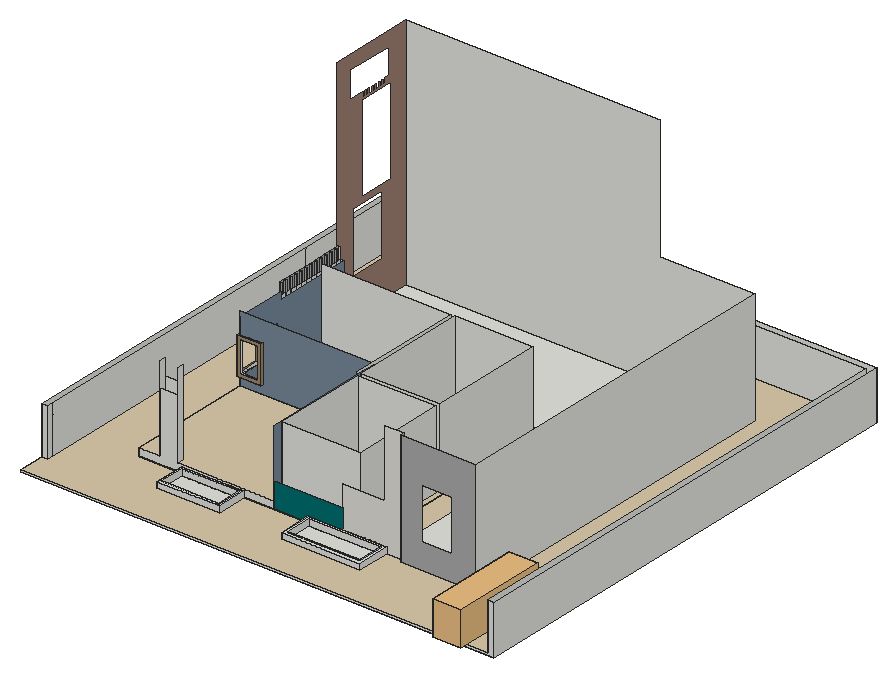
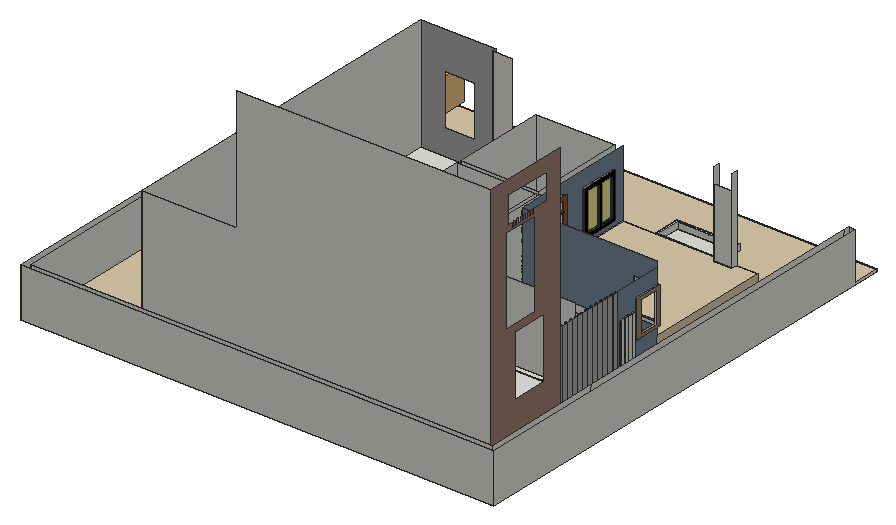
# SketchUp Ruby script. Lengths in inches.
U = 1.inch
M = Sketchup.active_model
def pt(a) = Geom::Point3d.new(a.map { |v| v * U })
def face(e, loops, mat)
  f = e.add_face(loops[0].map { |a| pt(a) })
  loops[1..].each { |l| e.add_face(l.map { |a| pt(a) }).erase! }
  f.material = f.back_material = mat if mat
  f
end
# faces: each face lists its corners as indices into pts; further lists are holes
def faces(e, pts, list, mat = nil) = list.each { |f| face(e, (f[0].is_a?(Array) ? f : [f]).map { |l| l.map { |i| pts[i] } }, mat) }
# xy, xz, yz: faces in a plane at the given z, y or x. An outline is a flat list of corners, or four numbers for a rectangle; further outlines are holes
def ring(l) = l.size == 4 ? [[l[0], l[1]], [l[2], l[1]], [l[2], l[3]], [l[0], l[3]]] : l.each_slice(2).to_a
def flat(e, list, mat, &to3) = list.each { |f| face(e, (f[0].is_a?(Array) ? f : [f]).map { |l| ring(l).map { |u, v| to3.(u, v) } }, mat) }
def xy(e, z, list, mat = nil) = flat(e, list, mat) { |x, y| [x, y, z] }
def xz(e, y, list, mat = nil) = flat(e, list, mat) { |x, z| [x, y, z] }
def yz(e, x, list, mat = nil) = flat(e, list, mat) { |y, z| [x, y, z] }
def lines(e, pts, list) = list.each { |a, b| e.add_line(pt(pts[a]), pt(pts[b])) }
# prism: a flat outline (further loops are holes) pulled along v
def prism(e, loops, v, mat = nil)
  f = face(e, loops, mat); d = Geom::Vector3d.new(v.map { |x| x * U })
  f.pushpull(f.normal.samedirection?(d) ? d.length : -d.length)
end
def box(e, o, s, mat = nil) = prism(e, [[o, [o[0] + s[0], o[1], o[2]], [o[0] + s[0], o[1] + s[1], o[2]], [o[0], o[1] + s[1], o[2]]]], [0, 0, s[2]], mat)
def at(x, y, z, deg = 0) = Geom::Transformation.translation(pt([x, y, z])) * Geom::Transformation.rotation(ORIGIN, Z_AXIS, deg.degrees)
def axes(o, x, y, z) = Geom::Transformation.new([*x, 0, *y, 0, *z, 0, *pt(o).to_a, 1])
def part(name) = M.definitions.add(name)
# library, detail: a bought-in or finely detailed component or shape, given as its bounding box
def library(name, o, s) = part(name).tap { |d| box(d.entities, o, s) }
def detail(e, o, s) = box(e.add_group.entities, o, s)
def put(e, d, t, mat = nil) = e.add_instance(d, t).tap { |i| i.material = mat if mat }
def group(e, t, mat = nil) = e.add_group.tap { |g| g.transformation = t; g.material = mat if mat }.entities
root = M.entities
M.materials.add("Niraj_Skin").color = [158, 128, 115]
M.materials.add("[0035_Tan]").color = [158, 135, 105]
M.materials.add("[0110_LightSlateGray]").color = [119, 136, 153]
M.materials.add("[Color H07]1").color = [0, 109, 109]
M.materials.add("[Color M03]").color = [170, 170, 170]
M.materials.add("[Color M09]").color = [0, 0, 0]
M.materials.add("[Field Square Tile]").color = [217, 201, 169]
M.materials.add("[Marble Carrara Gold Floor Tile]").color = [225, 223, 217]
M.materials.add("[Translucent Glass Gray]").color = [242, 225, 74]
M.materials["[Translucent Glass Gray]"].alpha = 0.5
M.materials.add("[Wood Cherry Original]").color = [152, 86, 42]
c1 = library("Potted plant collection",[-0.05,-0.05,0],[59.02,14.54,22.0625])
xy(root,12.61,[[[0,0,720.33,531.02],[89.54,112.91,428.79,458.91]],[89.54,112.91,89.54,266.1,98.54,266.1,98.54,121.91,294.79,121.91,294.79,112.91],[[294.79,112.91,294.79,266.1,89.54,266.1,89.54,458.91,428.79,458.91,428.79,112.91],[98.54,272.1,294.79,449.91],[300.79,272.1,419.79,449.91],[300.79,121.91,419.79,266.1]],[98.54,121.91,294.79,266.1],[300.79,121.91,419.79,266.1],
  [98.54,272.1,294.79,449.91],[300.79,272.1,419.79,449.91],[0,531.02,720.33,727.14]])
xy(root,15.11,[[98.54,121.91,98.54,305.6,294.79,305.6,294.79,286.89,288.79,286.89,288.79,280.89,291.79,280.89,291.79,260.11,288.79,260.11,288.79,257.5625,291.79,257.5625,291.79,233.45,288.79,233.45,288.79,227.45,294.79,227.45,294.79,121.91]])
xy(root,15.61,[[[347.53,62.1,467.15,112.91],[352.75,67.33,461.93,107.69]],[[154.8,66.73,250.05,112.91],[158.93,70.86,245.92,108.78]],[352.75,67.33,461.93,107.69],[158.93,70.86,245.92,108.78],[493.41,106.91,607.41,106.91,607.41,636.48,463.41,636.48,463.41,112.91,493.41,112.91],
  [294.79,112.91,428.79,112.91,428.79,458.91,89.54,458.91,89.54,305.6,294.79,305.6],[89.54,112.91,98.54,266.1],[98.54,112.91,121.875,121.91],[121.875,112.91,149.09,121.91],[149.09,112.91,294.79,121.91],
  [428.79,112.91,463.41,458.91],[288.79,227.45,294.79,233.45],[291.79,233.45,294.79,266.1],[288.79,257.5625,291.79,260.11],[89.54,266.1,98.54,305.6],
  [291.79,266.1,294.79,272.1],[291.79,272.1,294.79,280.89],[288.79,280.89,294.79,286.89],[86.54,350.68,89.54,354.7],[86.54,357.49,89.54,361.52],
  [86.54,364.68,89.54,368.7],[86.54,371.93,89.54,375.95],[89.54,458.91,463.41,458.91,463.41,636.48,77.54,636.48,77.54,504.04,89.54,504.04]])
xy(root,15.61,[[[0,0,711.33,0,711.33,718.14,9,718.14,9,40.8125,0,40.8125],[347.53,62.1,347.53,112.91,463.41,112.91,463.41,458.91,89.54,458.91,89.54,504.04,77.54,504.04,77.54,636.48,607.41,636.48,607.41,106.91,493.41,106.91,493.41,112.91,467.15,112.91,467.15,62.1],[154.8,66.73,250.05,112.91],[89.54,112.91,89.54,305.6,98.54,305.6,98.54,121.91,149.09,121.91,149.09,112.91],[81.04,392.11,84.04,398.71],[81.04,401.68,84.04,408.27],[81.04,411.24,84.04,417.84],[81.04,420.8,84.04,427.4],[81.04,430.36,84.04,436.96],[81.04,439.93,84.04,446.52],[81.04,449.49,84.04,456.09],[81.04,459.05,84.04,465.65],[81.04,468.61,84.04,475.21],[81.04,478.18,84.04,484.77],[81.04,487.86,84.04,494.46],[81.04,496.61,84.04,503.21],[86.54,350.68,89.54,354.7],[86.54,357.49,89.54,361.52],[86.54,364.68,89.54,368.7],[86.54,371.93,89.54,375.95]]],"[Field Square Tile]")
xy(root,23.13,[[288.79,233.45,291.79,257.5625],[288.79,260.11,291.79,280.89]])
xy(root,24.61,[[[347.53,62.1,467.15,112.91],[352.75,67.33,461.93,107.69]],[[154.8,66.73,250.05,112.91],[158.93,70.86,245.92,108.78]]])
xy(root,24.97,[[288.79,233.45,291.79,257.5625],[288.79,260.11,291.79,280.89]])
xy(root,27.61,[[89.54,112.91,121.875,112.91,121.875,121.91,149.09,121.91,149.09,112.91,294.79,112.91,294.79,227.45,288.79,227.45,288.79,233.45,291.79,233.45,291.79,257.5625,288.79,257.5625,288.79,260.11,291.79,260.11,291.79,280.89,288.79,280.89,288.79,286.89,294.79,286.89,294.79,305.6,89.54,305.6]],"[Field Square Tile]")
xy(root,36.97,[[291.79,131.57,294.79,189.85]])
xy(root,40.7,[[288.79,233.45,291.79,257.5625],[288.79,260.11,291.79,280.89]],"[Color M09]")
xy(root,40.99,[[86.54,302.6,86.54,346.85,89.54,346.85,89.54,305.6,123.91,305.6,123.91,302.6]])
xy(root,42.14,[[291.79,136.74,294.79,157.71],[291.79,160.71,294.79,184.67]],"[Color M09]")
xy(root,42.53,[[288.79,233.45,291.79,257.5625],[288.79,260.11,291.79,280.89]],"[Color M09]")
xz(root,0,[[0,12.61,720.33,12.61,720.33,87.61,711.33,87.61,711.33,15.61,0,15.61]])
xz(root,40.8125,[[0,15.61,9,87.61]])
xz(root,62.1,[[347.53,15.61,467.15,24.61]])
xz(root,66.73,[[154.8,15.61,250.05,24.61]])
xz(root,67.33,[[352.75,15.61,461.93,24.61]])
xz(root,70.86,[[158.93,15.61,245.92,24.61]])
xz(root,106.91,[[[493.41,15.61,607.41,188.93],[524.95,53.97,524.95,131.79,571.26,131.79,571.26,128.66,571.13,128.66,571.13,53.97]]],"[Color M03]")
xz(root,107.69,[[352.75,15.61,461.93,24.61]])
xz(root,108.78,[[158.93,15.61,245.92,24.61]])
xz(root,112.91,[[89.54,12.61,294.79,15.61],[294.79,12.61,428.79,15.61],[89.54,15.61,154.8,15.61,154.8,24.61,250.05,24.61,250.05,15.61,294.79,15.61,294.79,27.61,149.09,27.61,149.09,120.61,121.875,120.61,121.875,27.61,89.54,27.61],[154.8,15.61,250.05,24.61],[347.53,15.61,400.27,24.61],
  [400.27,15.61,428.79,24.61],[428.79,15.61,463.41,24.61],[463.41,15.61,467.15,24.61]])
xz(root,112.91,[[294.79,15.61,347.53,15.61,347.53,24.61,400.27,24.61,400.27,54.34,294.79,54.34]],"[Color H07]1")
xz(root,112.91,[[467.15,15.61,493.41,15.61,493.41,188.93,463.41,188.93,463.41,86.53,400.27,86.53,400.27,24.61,467.15,24.61]],"[Marble Carrara Gold Floor Tile]")
xz(root,121.91,[[98.54,12.61,121.875,15.11],[121.875,12.61,149.09,15.11],[149.09,12.61,294.79,15.11],[300.79,12.61,419.79,132.61],[98.54,15.11,121.875,15.61],
  [121.875,15.11,149.09,15.61],[149.09,15.11,294.79,15.61],[121.875,15.61,149.09,27.61],[121.875,27.61,149.09,132.61]])
xz(root,131.57,[[291.79,36.97,294.79,105.75]],"[Color M09]")
xz(root,136.74,[[291.79,42.14,294.79,100.57]],"[Color M09]")
xz(root,157.71,[[291.79,42.14,294.79,100.57]],"[Color M09]")
xz(root,160.71,[[291.79,42.14,294.79,100.57]],"[Color M09]")
xz(root,184.67,[[291.79,42.14,294.79,100.57]],"[Color M09]")
xz(root,189.85,[[291.79,36.97,294.79,105.75]],"[Color M09]")
xz(root,227.45,[[288.79,15.11,294.79,15.61],[288.79,15.61,294.79,27.61]])
xz(root,227.45,[[288.79,27.61,294.79,115.36]],"[Wood Cherry Original]")
xz(root,233.45,[[288.79,15.11,291.79,15.61],[288.79,15.61,291.79,23.13],[291.79,15.61,294.79,109.36],[288.79,23.13,291.79,24.97],[288.79,24.97,291.79,27.61],
  [288.79,40.7,291.79,42.53]])
xz(root,233.45,[[288.79,27.61,291.79,40.7],[288.79,42.53,291.79,58.26]],"[Wood Cherry Original]")
xz(root,257.5625,[[288.79,15.11,291.79,15.61],[288.79,15.61,291.79,23.13],[288.79,23.13,291.79,24.97],[288.79,24.97,291.79,27.61]])
xz(root,257.5625,[[288.79,42.53,291.79,58.26]],"[Color M09]")
xz(root,257.5625,[[288.79,27.61,291.79,40.7]],"[Wood Cherry Original]")
xz(root,260.11,[[288.79,15.11,291.79,15.61],[288.79,15.61,291.79,23.13],[288.79,23.13,291.79,24.97],[288.79,24.97,291.79,27.61]])
xz(root,260.11,[[288.79,27.61,291.79,40.7],[288.79,42.53,291.79,58.26]],"[Color M09]")
xz(root,266.1,[[300.79,12.61,419.79,132.61]])
xz(root,272.1,[[300.79,12.61,419.79,132.61]])
xz(root,280.89,[[288.79,15.11,291.79,15.61],[288.79,15.61,291.79,23.13],[291.79,15.61,294.79,109.36],[288.79,23.13,291.79,24.97],[288.79,24.97,291.79,27.61],
  [288.79,40.7,291.79,42.53]])
xz(root,280.89,[[288.79,27.61,291.79,40.7],[288.79,42.53,291.79,58.26]],"[Wood Cherry Original]")
xz(root,286.89,[[288.79,15.11,294.79,15.61],[288.79,15.61,294.79,27.61]])
xz(root,286.89,[[288.79,27.61,294.79,115.36]],"[Wood Cherry Original]")
xz(root,302.6,[[[86.54,40.99,123.91,97.01],[92.54,45.05,119.85,92.95]]],"[0035_Tan]")
xz(root,305.6,[[98.54,15.11,294.79,15.61],[89.54,15.61,294.79,27.61],[[89.54,40.99,123.91,97.01],[92.54,45.05,119.85,92.95]]])
xz(root,305.6,[[89.54,27.61,294.79,27.61,294.79,129.61,89.54,129.61,89.54,97.01,123.91,97.01,123.91,40.99,89.54,40.99]],"[0110_LightSlateGray]")
xz(root,346.85,[[86.54,40.99,89.54,97.01]])
xz(root,350.68,[[86.54,15.61,89.54,80.4]])
xz(root,354.7,[[86.54,15.61,89.54,80.4]])
xz(root,357.49,[[86.54,15.61,89.54,80.4]])
xz(root,361.52,[[86.54,15.61,89.54,80.4]])
xz(root,364.68,[[86.54,15.61,89.54,80.4]])
xz(root,368.7,[[86.54,15.61,89.54,80.4]])
xz(root,371.93,[[86.54,15.61,89.54,80.4]])
xz(root,375.95,[[86.54,15.61,89.54,80.4]])
xz(root,392.11,[[81.04,15.61,84.04,127.49]],"[Color M03]")
xz(root,398.71,[[81.04,15.61,84.04,127.49]],"[Color M03]")
xz(root,401.68,[[81.04,15.61,84.04,127.49]],"[Color M03]")
xz(root,408.27,[[81.04,15.61,84.04,127.49]],"[Color M03]")
xz(root,411.24,[[81.04,15.61,84.04,127.49]],"[Color M03]")
xz(root,417.84,[[81.04,15.61,84.04,127.49]],"[Color M03]")
xz(root,420.8,[[81.04,15.61,84.04,127.49]],"[Color M03]")
xz(root,427.4,[[81.04,15.61,84.04,127.49]],"[Color M03]")
xz(root,430.36,[[81.04,15.61,84.04,127.49]],"[Color M03]")
xz(root,436.96,[[81.04,15.61,84.04,127.49]],"[Color M03]")
xz(root,439.93,[[81.04,15.61,84.04,127.49]],"[Color M03]")
xz(root,446.52,[[81.04,15.61,84.04,127.49]],"[Color M03]")
xz(root,449.49,[[81.04,15.61,84.04,127.49]],"[Color M03]")
xz(root,449.91,[[98.54,12.61,294.79,132.61],[300.79,12.61,419.79,132.61]])
xz(root,456.09,[[81.04,15.61,84.04,127.49]],"[Color M03]")
xz(root,458.91,[[89.54,12.61,428.79,15.61]])
xz(root,459.05,[[81.04,15.61,84.04,127.49]],"[Color M03]")
xz(root,465.65,[[81.04,15.61,84.04,127.49]],"[Color M03]")
xz(root,468.61,[[81.04,15.61,84.04,127.49]],"[Color M03]")
xz(root,475.21,[[81.04,15.61,84.04,127.49]],"[Color M03]")
xz(root,478.18,[[81.04,15.61,84.04,127.49]],"[Color M03]")
xz(root,484.77,[[81.04,15.61,84.04,127.49]],"[Color M03]")
xz(root,487.86,[[81.04,15.61,84.04,127.49]],"[Color M03]")
xz(root,494.46,[[81.04,15.61,84.04,127.49]],"[Color M03]")
xz(root,496.61,[[81.04,15.61,84.04,127.49]],"[Color M03]")
xz(root,503.21,[[81.04,15.61,84.04,127.49]])
xz(root,504.04,[[77.54,15.61,89.54,110.36]])
xz(root,636.48,[[77.54,15.61,77.54,375.61,463.41,375.61,463.41,188.93,607.41,188.93,607.41,15.61]])
xz(root,718.14,[[9,15.61,711.33,87.61]])
xz(root,727.14,[[0,12.61,720.33,87.61]])
yz(root,0,[[0,12.61,0,15.61,40.8125,15.61,40.8125,87.61,727.14,87.61,727.14,12.61]])
yz(root,9,[[40.8125,15.61,49.8125,87.61],[49.8125,15.61,531.02,87.61],[531.02,15.61,718.14,87.61]])
yz(root,77.54,[[[504.04,15.61,636.48,375.61],[552.74,172.4,608.18,304.46],[536.21,70,591.21,162.875],[553.56,306.65,558.2,306.65,558.2,314.17,559.99,314.17,559.99,306.65,564.64,306.65,564.64,314.17,566.43,314.17,566.43,306.65,571.08,306.65,571.08,314.17,572.87,314.17,572.87,306.65,577.51,306.65,577.51,314.17,579.31,314.17,579.31,306.65,583.95,306.65,583.95,314.17,585.74,314.17,585.74,306.65,590.39,306.65,590.39,314.17,592.18,314.17,592.18,306.65,596.83,306.65,596.83,314.17,603.18,314.17,603.18,354.23,530.43,354.23,530.43,314.17,553.56,314.17]]],"Niraj_Skin")
yz(root,81.04,[[392.11,15.61,398.71,127.49],[401.68,15.61,408.27,127.49],[411.24,15.61,417.84,127.49],[420.8,15.61,427.4,127.49],[430.36,15.61,436.96,127.49],
  [439.93,15.61,446.52,127.49],[449.49,15.61,456.09,127.49],[459.05,15.61,465.65,127.49],[468.61,15.61,475.21,127.49],[478.18,15.61,484.77,127.49],
  [487.86,15.61,494.46,127.49],[496.61,15.61,503.21,127.49]],"[Color M03]")
yz(root,84.04,[[392.11,15.61,398.71,110.36],[401.68,15.61,408.27,110.36],[411.24,15.61,417.84,110.36],[420.8,15.61,427.4,110.36],[430.36,15.61,436.96,110.36],
  [439.93,15.61,446.52,110.36],[449.49,15.61,456.09,110.36],[459.05,15.61,465.65,110.36],[468.61,15.61,475.21,110.36],[478.18,15.61,484.77,110.36],
  [487.86,15.61,494.46,110.36],[496.61,15.61,503.21,110.36]])
yz(root,86.54,[[350.68,15.61,354.7,80.4],[357.49,15.61,361.52,80.4],[364.68,15.61,368.7,80.4],[371.93,15.61,375.95,80.4]])
yz(root,86.54,[[[302.6,40.99,346.85,97.01],[308.6,45.39,339.85,92.95]]],"[0035_Tan]")
yz(root,89.54,[[112.91,12.61,266.1,15.61],[266.1,12.61,458.91,15.61],[350.68,15.61,354.7,80.4],[357.49,15.61,361.52,80.4],[364.68,15.61,368.7,80.4],
  [371.93,15.61,375.95,80.4],[305.6,40.99,342.85,42.39],[[342.85,40.99,346.85,40.99,346.85,97.01,305.6,97.01,305.6,42.39,342.85,42.39],[308.6,45.39,339.85,92.95]]])
yz(root,89.54,[[305.6,15.61,305.6,40.99,346.85,40.99,346.85,97.01,305.6,97.01,305.6,120.61,383.99,120.61,383.99,110.36,504.04,110.36,504.04,15.61,375.95,15.61,375.95,80.4,371.93,80.4,371.93,15.61,368.7,15.61,368.7,80.4,364.68,80.4,364.68,15.61,361.52,15.61,361.52,80.4,357.49,80.4,357.49,15.61,354.7,15.61,354.7,80.4,350.68,80.4,350.68,15.61]],"[0110_LightSlateGray]")
yz(root,89.54,[[112.91,15.61,305.6,27.61]],"[Field Square Tile]")
yz(root,98.54,[[121.91,12.61,266.1,15.11],[272.1,12.61,305.6,15.11],[121.91,15.11,266.1,15.61],[266.1,15.11,272.1,15.61],[272.1,15.11,305.6,15.61]])
yz(root,121.875,[[112.91,27.61,121.91,156.61]])
yz(root,123.91,[[302.6,40.99,305.6,97.01]],"[0035_Tan]")
yz(root,149.09,[[112.91,27.61,121.91,156.61]])
yz(root,154.8,[[66.73,15.61,112.91,24.61]])
yz(root,158.93,[[70.86,15.61,108.78,24.61]])
yz(root,245.92,[[70.86,15.61,108.78,24.61]])
yz(root,250.05,[[66.73,15.61,112.91,24.61]])
yz(root,288.79,[[227.45,15.11,233.45,15.61],[257.5625,15.11,260.11,15.61],[280.89,15.11,286.89,15.61],[227.45,15.61,233.45,27.61],[257.5625,15.61,260.11,27.61],
  [280.89,15.61,286.89,27.61],[233.45,23.13,257.5625,24.97],[260.11,23.13,280.89,24.97]])
yz(root,288.79,[[257.5625,27.61,257.5625,40.7,233.45,40.7,233.45,42.53,257.5625,42.53,257.5625,58.26,233.45,58.26,233.45,60.09,257.5625,60.09,257.5625,75.82,233.45,75.82,233.45,77.65,257.5625,77.65,257.5625,93.38,233.45,93.38,233.45,95.22,257.5625,95.22,257.5625,109.36,260.11,109.36,260.11,95.22,280.89,95.22,280.89,93.38,260.11,93.38,260.11,77.65,280.89,77.65,280.89,75.82,260.11,75.82,260.11,60.09,280.89,60.09,280.89,58.26,260.11,58.26,260.11,42.53,280.89,42.53,280.89,40.7,260.11,40.7,260.11,27.61]],"[Color M09]")
yz(root,288.79,[[227.45,27.61,227.45,115.36,286.89,115.36,286.89,27.61,280.89,27.61,280.89,109.36,233.45,109.36,233.45,27.61]],"[Wood Cherry Original]")
yz(root,291.79,[[233.45,15.11,257.5625,15.61],[260.11,15.11,266.1,15.61],[266.1,15.11,272.1,15.61],[272.1,15.11,280.89,15.61],[233.45,15.61,257.5625,23.13],
  [257.5625,15.61,260.11,15.61,260.11,40.7,280.89,40.7,280.89,42.53,260.11,42.53,260.11,58.26,280.89,58.26,280.89,60.09,260.11,60.09,260.11,75.82,280.89,75.82,280.89,77.65,260.11,77.65,260.11,93.38,280.89,93.38,280.89,95.22,260.11,95.22,260.11,109.36,257.5625,109.36,257.5625,95.22,233.45,95.22,233.45,93.38,257.5625,93.38,257.5625,77.65,233.45,77.65,233.45,75.82,257.5625,75.82,257.5625,60.09,233.45,60.09,233.45,58.26,257.5625,58.26,257.5625,42.53,233.45,42.53,233.45,40.7,257.5625,40.7],[260.11,15.61,266.1,23.13],[266.1,15.61,272.1,23.13],[272.1,15.61,280.89,23.13],[233.45,23.13,257.5625,24.97],
  [260.11,23.13,266.1,24.97],[266.1,23.13,272.1,24.97],[272.1,23.13,280.89,24.97],[233.45,24.97,257.5625,27.61],[260.11,24.97,266.1,27.61],
  [266.1,24.97,272.1,27.61],[272.1,24.97,280.89,27.61]])
yz(root,291.79,[[[131.57,36.97,189.85,105.75],[160.71,42.14,184.67,100.57],[136.74,42.14,157.71,100.57]]],"[Color M09]")
yz(root,291.79,[[233.45,27.61,257.5625,40.7],[260.11,27.61,280.89,40.7],[233.45,42.53,257.5625,58.26],[260.11,42.53,280.89,58.26]],"[Translucent Glass Gray]")
yz(root,294.79,[[112.91,12.61,121.91,15.61],[121.91,12.61,227.45,15.11],[227.45,12.61,266.1,15.61],[272.1,12.61,286.89,15.61],[305.6,12.61,305.6,129.61,272.1,129.61,272.1,132.61,449.91,132.61,449.91,12.61],
  [286.89,12.61,305.6,15.11],[121.91,15.11,227.45,15.61],[286.89,15.11,305.6,15.61],[112.91,15.61,227.45,27.61],[227.45,15.61,233.45,15.61,233.45,109.36,280.89,109.36,280.89,15.61,286.89,15.61,286.89,115.36,227.45,115.36],
  [286.89,15.61,305.6,27.61],[[131.57,36.97,189.85,105.75],[160.71,42.14,184.67,100.57],[136.74,42.14,157.71,100.57]]])
yz(root,294.79,[[[112.91,27.61,112.91,129.61,305.6,129.61,305.6,27.61,286.89,27.61,286.89,115.36,227.45,115.36,227.45,27.61],[131.57,36.97,189.85,105.75]]],"[0110_LightSlateGray]")
yz(root,294.79,[[136.74,42.14,157.71,100.57],[160.71,42.14,184.67,100.57]],"[Translucent Glass Gray]")
yz(root,300.79,[[121.91,12.61,266.1,132.61],[272.1,12.61,449.91,132.61]])
yz(root,347.53,[[62.1,15.61,112.91,24.61]])
yz(root,352.75,[[67.33,15.61,107.69,24.61]])
yz(root,419.79,[[121.91,12.61,266.1,132.61],[272.1,12.61,449.91,132.61]])
yz(root,428.79,[[112.91,12.61,458.91,15.61]])
yz(root,461.93,[[67.33,15.61,107.69,24.61]])
yz(root,467.15,[[62.1,15.61,112.91,24.61]])
yz(root,493.41,[[106.91,15.61,112.91,188.93]],"[Color M03]")
yz(root,607.41,[[106.91,15.61,636.48,188.93]])
yz(root,711.33,[[0,15.61,718.14,87.61]])
yz(root,720.33,[[0,12.61,727.14,87.61]])
p = [[89.54,305.6,42.39],[86.54,305.6,42.39],[291.79,266.1,12.61],[291.79,266.1,15.11],[291.79,272.1,12.61],[291.79,272.1,15.11]]
lines(root,p,[[0,1],[2,3],[4,5]])
put(root,c1,axes([635.03,135.78,15.61],[0,-2.47629,0],[2.96687,0,0],[0,0,2.33612]))
